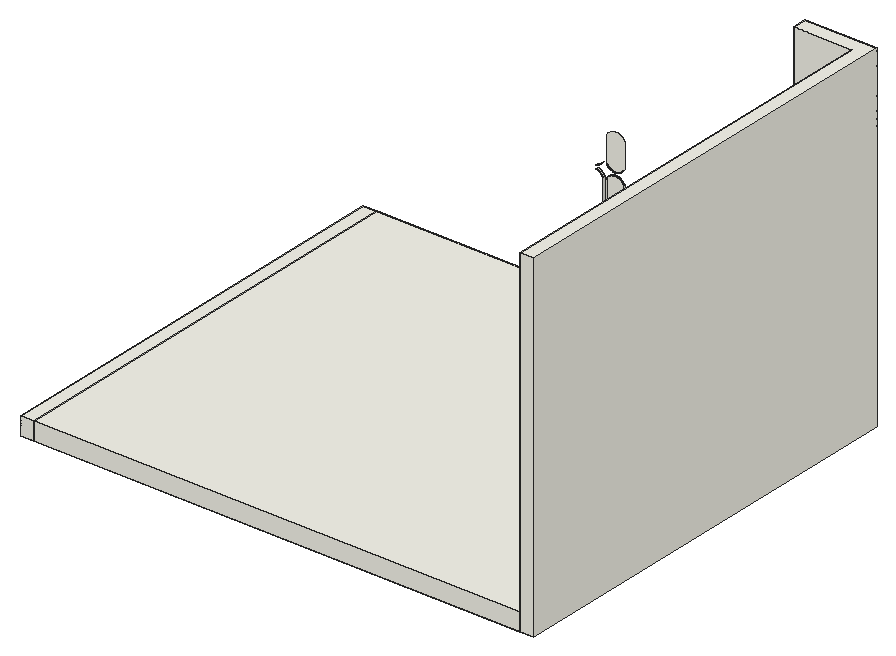
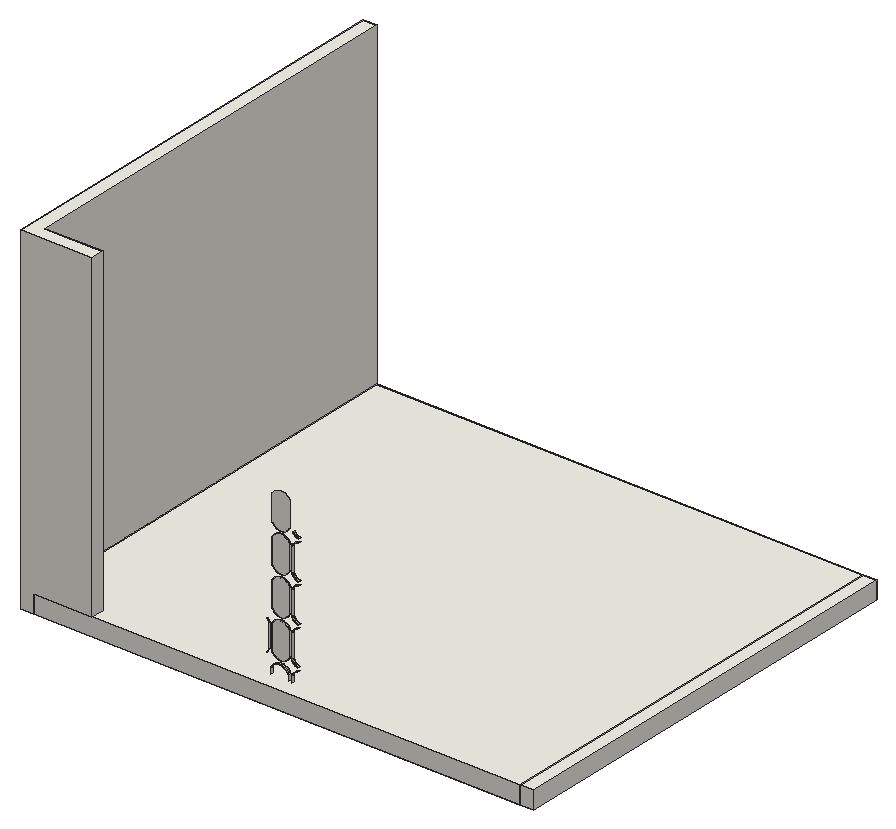
# SketchUp Ruby script. Lengths in inches.
U = 1.inch
M = Sketchup.active_model
def pt(a) = Geom::Point3d.new(a.map { |v| v * U })
def face(e, loops, mat)
  f = e.add_face(loops[0].map { |a| pt(a) })
  loops[1..].each { |l| e.add_face(l.map { |a| pt(a) }).erase! }
  f.material = f.back_material = mat if mat
  f
end
# faces: each face lists its corners as indices into pts; further lists are holes
def faces(e, pts, list, mat = nil) = list.each { |f| face(e, (f[0].is_a?(Array) ? f : [f]).map { |l| l.map { |i| pts[i] } }, mat) }
# xy, xz, yz: faces in a plane at the given z, y or x. An outline is a flat list of corners, or four numbers for a rectangle; further outlines are holes
def ring(l) = l.size == 4 ? [[l[0], l[1]], [l[2], l[1]], [l[2], l[3]], [l[0], l[3]]] : l.each_slice(2).to_a
def flat(e, list, mat, &to3) = list.each { |f| face(e, (f[0].is_a?(Array) ? f : [f]).map { |l| ring(l).map { |u, v| to3.(u, v) } }, mat) }
def xy(e, z, list, mat = nil) = flat(e, list, mat) { |x, y| [x, y, z] }
def xz(e, y, list, mat = nil) = flat(e, list, mat) { |x, z| [x, y, z] }
def yz(e, x, list, mat = nil) = flat(e, list, mat) { |y, z| [x, y, z] }
def lines(e, pts, list) = list.each { |a, b| e.add_line(pt(pts[a]), pt(pts[b])) }
# prism: a flat outline (further loops are holes) pulled along v
def prism(e, loops, v, mat = nil)
  f = face(e, loops, mat); d = Geom::Vector3d.new(v.map { |x| x * U })
  f.pushpull(f.normal.samedirection?(d) ? d.length : -d.length)
end
def box(e, o, s, mat = nil) = prism(e, [[o, [o[0] + s[0], o[1], o[2]], [o[0] + s[0], o[1] + s[1], o[2]], [o[0], o[1] + s[1], o[2]]]], [0, 0, s[2]], mat)
def at(x, y, z, deg = 0) = Geom::Transformation.translation(pt([x, y, z])) * Geom::Transformation.rotation(ORIGIN, Z_AXIS, deg.degrees)
def axes(o, x, y, z) = Geom::Transformation.new([*x, 0, *y, 0, *z, 0, *pt(o).to_a, 1])
def part(name) = M.definitions.add(name)
# library, detail: a bought-in or finely detailed component or shape, given as its bounding box
def library(name, o, s) = part(name).tap { |d| box(d.entities, o, s) }
def detail(e, o, s) = box(e.add_group.entities, o, s)
def put(e, d, t, mat = nil) = e.add_instance(d, t).tap { |i| i.material = mat if mat }
def group(e, t, mat = nil) = e.add_group.tap { |g| g.transformation = t; g.material = mat if mat }.entities
root = M.entities
M.materials.add("Tafisa-Gardenia-or-Gardenia-PM775-4K").color = [246, 245, 235]
xz(root,138.25,[[89.53,11,89.85,11.02,90.17,11.0625,90.48,11.14,90.78,11.25,91.07,11.38,91.35,11.55,91.61,11.73,91.84,11.95,92.0625,12.18,92.25,12.4375,92.42,12.71,92.5625,13,92.5625,21,92.42,21.29,92.25,21.5625,92.0625,21.82,91.84,22.05,91.61,22.27,91.35,22.45,91.07,22.62,90.78,22.75,90.48,22.86,90.17,22.9375,89.85,22.98,89.53,23,89.21,22.98,89.02,22.96,88.89,22.9375,88.58,22.86,88.28,22.75,87.99,22.62,87.72,22.45,87.46,22.27,87.22,22.05,87,21.82,86.81,21.5625,86.64,21.29,86.5,21,86.5,13,86.64,12.71,86.81,12.4375,87,12.18,87.22,11.95,87.46,11.73,87.72,11.55,87.99,11.38,88.28,11.25,88.58,11.14,88.89,11.0625,89.21,11.02],[89.53,24,89.85,24.02,90.17,24.0625,90.48,24.14,90.78,24.25,91.07,24.38,91.35,24.55,91.61,24.73,91.84,24.95,92.0625,25.18,92.25,25.4375,92.42,25.71,92.5625,26,92.5625,34,92.42,34.29,92.25,34.5625,92.0625,34.82,91.84,35.05,91.61,35.27,91.35,35.45,91.07,35.62,90.78,35.75,90.48,35.86,90.17,35.9375,89.85,35.98,89.53,36,89.21,35.98,89.02,35.96,88.89,35.9375,88.58,35.86,88.28,35.75,87.99,35.62,87.72,35.45,87.46,35.27,87.22,35.05,87,34.82,86.86,34.63,86.81,34.5625,86.64,34.29,86.5,34,86.5,26,86.64,25.71,86.81,25.4375,87,25.18,87.22,24.95,87.46,24.73,87.72,24.55,87.99,24.38,88.28,24.25,88.58,24.14,88.89,24.0625,89.02,24.04,89.21,24.02],[89.53,37,89.85,37.02,90.17,37.0625,90.48,37.14,90.78,37.25,91.07,37.38,91.35,37.55,91.61,37.73,91.84,37.95,92.0625,38.18,92.25,38.4375,92.42,38.71,92.5625,39,92.5625,47,92.42,47.29,92.25,47.5625,92.0625,47.82,91.84,48.05,91.61,48.27,91.35,48.45,91.07,48.62,90.78,48.75,90.48,48.86,90.17,48.9375,89.85,48.98,89.53,49,89.21,48.98,89.02,48.96,88.89,48.9375,88.58,48.86,88.28,48.75,87.99,48.62,87.72,48.45,87.46,48.27,87.22,48.05,87,47.82,86.81,47.5625,86.64,47.29,86.5,47,86.5,39,86.64,38.71,86.81,38.4375,87,38.18,87.22,37.95,87.46,37.73,87.72,37.55,87.99,37.38,88.28,37.25,88.58,37.14,88.89,37.0625,89.02,37.04,89.21,37.02],[89.53,50,89.85,50.02,90.17,50.0625,90.48,50.14,90.78,50.25,91.07,50.38,91.35,50.55,91.61,50.73,91.84,50.95,92.0625,51.18,92.25,51.4375,92.42,51.71,92.5625,52,92.5625,60,92.42,60.29,92.25,60.5625,92.0625,60.82,91.84,61.05,91.61,61.27,91.35,61.45,91.07,61.62,90.78,61.75,90.48,61.86,90.17,61.9375,89.85,61.98,89.53,62,89.21,61.98,89.02,61.96,88.89,61.9375,88.58,61.86,88.28,61.75,87.99,61.62,87.72,61.45,87.46,61.27,87.22,61.05,87,60.82,86.81,60.5625,86.64,60.29,86.5,60,86.5,52,86.64,51.71,86.81,51.4375,87,51.18,87.22,50.95,87.46,50.73,87.72,50.55,87.99,50.38,88.28,50.25,88.58,50.14,88.89,50.0625,89.02,50.04,89.21,50.02]],"Tafisa-Gardenia-or-Gardenia-PM775-4K")
yz(root,85.5,[[138,6,138.79,8],[138,13,138.79,21],[138,26,138.79,34],[138,39,138.79,47]])
yz(root,86.5,[[138,6,138.79,8]])
yz(root,86.5,[[138,13,138.25,21],[138,26,138.25,34],[138,39,138.25,47]],"Tafisa-Gardenia-or-Gardenia-PM775-4K")
yz(root,92.5625,[[138,6,138.79,8]])
yz(root,92.5625,[[138,13,138.25,21],[138,26,138.25,34],[138,39,138.25,47]],"Tafisa-Gardenia-or-Gardenia-PM775-4K")
yz(root,93.5625,[[138,13,138.25,21]],"Tafisa-Gardenia-or-Gardenia-PM775-4K")
p = [[85.36,138.79,8.29],[85.5,138.79,8],[85.5,138,8],[85.36,138,8.29],[86.5,138.79,8],[86.64,138.79,8.29],
  [86.64,138,8.29],[86.5,138,8],[92.42,138.79,8.29],[92.5625,138.79,8],[92.5625,138,8],[92.42,138,8.29],
  [85.2,138.79,8.56],[85.2,138,8.56],[86.81,138.79,8.5625],[86.81,138,8.5625],[92.25,138.79,8.5625],[92.25,138,8.5625],
  [85.01,138.79,8.82],[85.01,138,8.82],[87,138.79,8.82],[87,138,8.82],[92.0625,138.79,8.82],[92.0625,138,8.82],
  [84.79,138.79,9.05],[84.79,138,9.05],[87.22,138.79,9.05],[87.22,138,9.05],[91.84,138.79,9.05],[91.84,138,9.05],
  [84.56,138.79,9.26],[84.56,138,9.26],[87.46,138.79,9.27],[87.46,138,9.27],[91.61,138.79,9.27],[91.61,138,9.27],
  [84.3,138.79,9.45],[84.3,138,9.45],[87.72,138.79,9.45],[87.72,138,9.45],[91.35,138.79,9.45],[91.35,138,9.45],
  [84.03,138.79,9.62],[84.03,138,9.62],[87.99,138.79,9.62],[87.99,138,9.62],[91.07,138.79,9.62],[91.07,138,9.62],
  [83.74,138.79,9.75],[83.74,138,9.75],[88.28,138.79,9.75],[88.28,138,9.75],[90.78,138.79,9.75],[90.78,138,9.75],
  [83.44,138.79,9.86],[83.44,138,9.86],[88.58,138.79,9.86],[88.58,138,9.86],[90.48,138.79,9.86],[90.48,138,9.86],
  [88.89,138.79,9.9375],[88.89,138,9.9375],[89.21,138.79,9.98],[89.21,138,9.98],[89.85,138.79,9.98],[90.17,138.79,9.9375],
  [90.17,138,9.9375],[89.85,138,9.98],[89.53,138.79,10],[89.53,138,10],[88.89,138,11.0625],[89.21,138,11.02],
  [89.21,138.25,11.02],[88.89,138.25,11.0625],[89.53,138,11],[89.53,138.25,11],[89.85,138,11.02],[89.85,138.25,11.02],
  [90.17,138,11.0625],[90.17,138.25,11.0625],[83.74,138.79,11.25],[83.44,138.79,11.14],[83.44,138,11.14],[83.74,138,11.25],
  [88.28,138,11.25],[88.58,138,11.14],[88.58,138.25,11.14],[88.28,138.25,11.25],[90.48,138,11.14],[90.48,138.25,11.14],
  [90.78,138,11.25],[90.78,138.25,11.25],[84.03,138.79,11.38],[84.03,138,11.38],[87.99,138,11.38],[87.99,138.25,11.38],
  [91.07,138,11.38],[91.07,138.25,11.38],[84.3,138.79,11.55],[84.3,138,11.55],[87.72,138,11.55],[87.72,138.25,11.55],
  [91.35,138,11.55],[91.35,138.25,11.55],[84.56,138.79,11.74],[84.56,138,11.74],[87.46,138,11.73],[87.46,138.25,11.73],
  [91.61,138,11.73],[91.61,138.25,11.73],[84.79,138.79,11.95],[84.79,138,11.95],[87.22,138,11.95],[87.22,138.25,11.95],
  [91.84,138,11.95],[91.84,138.25,11.95],[85.01,138.79,12.18],[85.01,138,12.18],[87,138,12.18],[87,138.25,12.18],
  [92.0625,138,12.18],[92.0625,138.25,12.18],[94.04,138,12.19],[94.25,138,11.95],[94.25,138.25,11.95],[94.04,138.25,12.19],
  [85.2,138.79,12.44],[85.2,138,12.44],[86.81,138,12.4375],[86.81,138.25,12.4375],[92.25,138,12.4375],[92.25,138.25,12.4375],
  [93.86,138,12.44],[93.86,138.25,12.44],[85.36,138.79,12.71],[85.36,138,12.71],[86.64,138,12.71],[86.64,138.25,12.71],
  [92.42,138,12.71],[92.42,138.25,12.71],[93.7,138,12.71],[93.7,138.25,12.71],[85.5,138.79,13],[85.5,138,13],
  [86.5,138,13],[86.5,138.25,13],[92.5625,138,13],[92.5625,138.25,13],[93.5625,138,13],[93.5625,138.25,13],
  [85.36,138.79,21.29],[85.5,138.79,21],[85.5,138,21],[85.36,138,21.29],[86.64,138,21.29],[86.5,138,21],
  [86.5,138.25,21],[86.64,138.25,21.29],[92.5625,138,21],[92.42,138,21.29],[92.42,138.25,21.29],[92.5625,138.25,21],
  [93.7,138,21.29],[93.5625,138,21],[93.5625,138.25,21],[93.7,138.25,21.29],[85.2,138.79,21.56],[85.2,138,21.56],
  [86.81,138,21.5625],[86.81,138.25,21.5625],[92.25,138,21.5625],[92.25,138.25,21.5625],[93.86,138,21.56],[93.86,138.25,21.56],
  [85.01,138.79,21.82],[85.01,138,21.82],[87,138,21.82],[87,138.25,21.82],[92.0625,138,21.82],[92.0625,138.25,21.82],
  [94.04,138,21.81],[94.04,138.25,21.81],[84.79,138.79,22.05],[84.79,138,22.05],[87.22,138,22.05],[87.22,138.25,22.05],
  [91.84,138,22.05],[91.84,138.25,22.05],[94.25,138,22.05],[94.25,138.25,22.05],[84.56,138.79,22.26],[84.56,138,22.26],
  [87.46,138,22.27],[87.46,138.25,22.27],[91.61,138,22.27],[91.61,138.25,22.27],[84.3,138.79,22.45],[84.3,138,22.45],
  [87.72,138,22.45],[87.72,138.25,22.45],[91.35,138,22.45],[91.35,138.25,22.45],[84.03,138.79,22.62],[84.03,138,22.62],
  [87.99,138,22.62],[87.99,138.25,22.62],[91.07,138,22.62],[91.07,138.25,22.62],[83.74,138.79,22.75],[83.74,138,22.75],
  [88.28,138,22.75],[88.28,138.25,22.75],[90.78,138,22.75],[90.78,138.25,22.75],[83.44,138.79,22.86],[83.44,138,22.86],
  [88.58,138,22.86],[88.58,138.25,22.86],[90.48,138,22.86],[90.48,138.25,22.86],[88.89,138,22.9375],[88.89,138.25,22.9375],
  [89.02,138,22.96],[89.02,138.25,22.96],[90.17,138,22.9375],[89.85,138,22.98],[89.85,138.25,22.98],[90.17,138.25,22.9375],
  [89.21,138,22.98],[89.21,138.25,22.98],[89.53,138,23],[89.53,138.25,23],[88.89,138,24.0625],[89.02,138,24.04],
  [89.02,138.25,24.04],[88.89,138.25,24.0625],[89.21,138,24.02],[89.21,138.25,24.02],[89.53,138,24],[89.53,138.25,24],
  [89.85,138,24.02],[89.85,138.25,24.02],[90.17,138,24.0625],[90.17,138.25,24.0625],[83.44,138.79,24.14],[83.13,138.79,24.0625],
  [83.13,138,24.0625],[83.44,138,24.14],[83.74,138.79,24.25],[83.74,138,24.25],[88.28,138,24.25],[88.58,138,24.14],
  [88.58,138.25,24.14],[88.28,138.25,24.25],[90.48,138,24.14],[90.48,138.25,24.14],[90.78,138,24.25],[90.78,138.25,24.25],
  [84.03,138.79,24.38],[84.03,138,24.38],[87.99,138,24.38],[87.99,138.25,24.38],[91.07,138,24.38],[91.07,138.25,24.38],
  [84.3,138.79,24.55],[84.3,138,24.55],[87.72,138,24.55],[87.72,138.25,24.55],[91.35,138,24.55],[91.35,138.25,24.55],
  [84.56,138.79,24.74],[84.56,138,24.74],[87.46,138,24.73],[87.46,138.25,24.73],[91.61,138,24.73],[91.61,138.25,24.73],
  [84.79,138.79,24.95],[84.79,138,24.95],[87.22,138,24.95],[87.22,138.25,24.95],[91.84,138,24.95],[91.84,138.25,24.95],
  [85.01,138.79,25.18],[85.01,138,25.18],[87,138,25.18],[87,138.25,25.18],[92.0625,138,25.18],[92.0625,138.25,25.18],
  [85.2,138.79,25.44],[85.2,138,25.44],[86.81,138,25.4375],[86.81,138.25,25.4375],[92.25,138,25.4375],[92.25,138.25,25.4375],
  [85.36,138.79,25.71],[85.36,138,25.71],[86.64,138,25.71],[86.64,138.25,25.71],[92.42,138,25.71],[92.42,138.25,25.71],
  [85.5,138.79,26],[85.5,138,26],[86.5,138,26],[86.5,138.25,26],[92.5625,138,26],[92.5625,138.25,26],
  [85.36,138.79,34.29],[85.5,138.79,34],[85.5,138,34],[85.36,138,34.29],[86.64,138,34.29],[86.5,138,34],
  [86.5,138.25,34],[86.64,138.25,34.29],[92.5625,138,34],[92.42,138,34.29],[92.42,138.25,34.29],[92.5625,138.25,34],
  [85.2,138.79,34.56],[85.2,138,34.56],[86.81,138,34.5625],[86.81,138.25,34.5625],[92.25,138,34.5625],[92.25,138.25,34.5625],
  [85.01,138.79,34.82],[85.01,138,34.82],[86.86,138,34.63],[86.86,138.25,34.63],[87,138,34.82],[87,138.25,34.82],
  [92.0625,138,34.82],[92.0625,138.25,34.82],[84.79,138.79,35.05],[84.79,138,35.05],[87.22,138,35.05],[87.22,138.25,35.05],
  [91.84,138,35.05],[91.84,138.25,35.05],[84.56,138.79,35.26],[84.56,138,35.26],[87.46,138,35.27],[87.46,138.25,35.27],
  [91.61,138,35.27],[91.61,138.25,35.27],[84.3,138.79,35.45],[84.3,138,35.45],[87.72,138,35.45],[87.72,138.25,35.45],
  [91.35,138,35.45],[91.35,138.25,35.45],[84.03,138.79,35.62],[84.03,138,35.62],[87.99,138,35.62],[87.99,138.25,35.62],
  [91.07,138,35.62],[91.07,138.25,35.62],[83.74,138.79,35.75],[83.74,138,35.75],[88.28,138,35.75],[88.28,138.25,35.75],
  [90.78,138,35.75],[90.78,138.25,35.75],[83.44,138.79,35.86],[83.44,138,35.86],[88.58,138,35.86],[88.58,138.25,35.86],
  [90.48,138,35.86],[90.48,138.25,35.86],[83.13,138.79,35.9375],[83.13,138,35.9375],[88.89,138,35.9375],[88.89,138.25,35.9375],
  [89.02,138,35.96],[89.02,138.25,35.96],[90.17,138,35.9375],[89.85,138,35.98],[89.85,138.25,35.98],[90.17,138.25,35.9375],
  [89.21,138,35.98],[89.21,138.25,35.98],[89.53,138,36],[89.53,138.25,36],[88.89,138,37.0625],[89.02,138,37.04],
  [89.02,138.25,37.04],[88.89,138.25,37.0625],[89.21,138,37.02],[89.21,138.25,37.02],[89.53,138,37],[89.53,138.25,37],
  [89.85,138,37.02],[89.85,138.25,37.02],[90.17,138,37.0625],[90.17,138.25,37.0625],[83.44,138.79,37.14],[83.13,138.79,37.0625],
  [83.13,138,37.0625],[83.44,138,37.14],[83.74,138.79,37.25],[83.74,138,37.25],[88.28,138,37.25],[88.58,138,37.14],
  [88.58,138.25,37.14],[88.28,138.25,37.25],[90.48,138,37.14],[90.48,138.25,37.14],[90.78,138,37.25],[90.78,138.25,37.25],
  [84.03,138.79,37.38],[84.03,138,37.38],[87.99,138,37.38],[87.99,138.25,37.38],[91.07,138,37.38],[91.07,138.25,37.38],
  [84.3,138.79,37.55],[84.3,138,37.55],[87.72,138,37.55],[87.72,138.25,37.55],[91.35,138,37.55],[91.35,138.25,37.55],
  [84.46,138,37.66],[84.46,138.79,37.66],[87.46,138,37.73],[87.46,138.25,37.73],[91.61,138,37.73],[91.61,138.25,37.73],
  [84.56,138.79,37.74],[84.56,138,37.74],[84.79,138.79,37.95],[84.79,138,37.95],[87.22,138,37.95],[87.22,138.25,37.95],
  [91.84,138,37.95],[91.84,138.25,37.95],[85.01,138.79,38.18],[85.01,138,38.18],[87,138,38.18],[87,138.25,38.18],
  [92.0625,138,38.18],[92.0625,138.25,38.18],[85.2,138.79,38.44],[85.2,138,38.44],[86.81,138,38.4375],[86.81,138.25,38.4375],
  [92.25,138,38.4375],[92.25,138.25,38.4375],[85.36,138.79,38.71],[85.36,138,38.71],[86.64,138,38.71],[86.64,138.25,38.71],
  [92.42,138,38.71],[92.42,138.25,38.71],[85.5,138.79,39],[85.5,138,39],[86.5,138,39],[86.5,138.25,39],
  [92.5625,138,39],[92.5625,138.25,39],[85.36,138.79,47.29],[85.5,138.79,47],[85.5,138,47],[85.36,138,47.29],
  [86.64,138,47.29],[86.5,138,47],[86.5,138.25,47],[86.64,138.25,47.29],[92.5625,138,47],[92.42,138,47.29],
  [92.42,138.25,47.29],[92.5625,138.25,47],[85.2,138.79,47.56],[85.2,138,47.56],[86.81,138,47.5625],[86.81,138.25,47.5625],
  [92.25,138,47.5625],[92.25,138.25,47.5625],[85.01,138.79,47.82],[85.01,138,47.82],[87,138,47.82],[87,138.25,47.82],
  [92.0625,138,47.82],[92.0625,138.25,47.82],[84.79,138.79,48.05],[84.79,138,48.05],[87.22,138,48.05],[87.22,138.25,48.05],
  [91.84,138,48.05],[91.84,138.25,48.05],[84.56,138.79,48.26],[84.56,138,48.26],[87.46,138,48.27],[87.46,138.25,48.27],
  [91.61,138,48.27],[91.61,138.25,48.27],[84.3,138.79,48.45],[84.3,138,48.45],[87.72,138,48.45],[87.72,138.25,48.45],
  [91.35,138,48.45],[91.35,138.25,48.45],[84.03,138.79,48.62],[84.03,138,48.62],[87.99,138,48.62],[87.99,138.25,48.62],
  [91.07,138,48.62],[91.07,138.25,48.62],[83.74,138.79,48.75],[83.74,138,48.75],[88.28,138,48.75],[88.28,138.25,48.75],
  [90.78,138,48.75],[90.78,138.25,48.75],[83.44,138.79,48.86],[83.44,138,48.86],[88.58,138,48.86],[88.58,138.25,48.86],
  [90.48,138,48.86],[90.48,138.25,48.86],[83.13,138.79,48.9375],[83.13,138,48.9375],[88.89,138,48.9375],[88.89,138.25,48.9375],
  [89.02,138,48.96],[89.02,138.25,48.96],[90.17,138,48.9375],[89.85,138,48.98],[89.85,138.25,48.98],[90.17,138.25,48.9375],
  [89.21,138,48.98],[89.21,138.25,48.98],[89.53,138,49],[89.53,138.25,49],[88.89,138,50.0625],[89.02,138,50.04],
  [89.02,138.25,50.04],[88.89,138.25,50.0625],[89.21,138,50.02],[89.21,138.25,50.02],[89.53,138,50],[89.53,138.25,50],
  [89.85,138,50.02],[89.85,138.25,50.02],[90.17,138,50.0625],[90.17,138.25,50.0625],[83.44,138.79,50.14],[83.13,138.79,50.0625],
  [83.13,138,50.0625],[83.44,138,50.14],[83.74,138.79,50.25],[83.74,138,50.25],[88.28,138,50.25],[88.58,138,50.14],
  [88.58,138.25,50.14],[88.28,138.25,50.25],[90.48,138,50.14],[90.48,138.25,50.14],[90.78,138,50.25],[90.78,138.25,50.25],
  [84.03,138.79,50.38],[84.03,138,50.38],[87.99,138,50.38],[87.99,138.25,50.38],[91.07,138,50.38],[91.07,138.25,50.38],
  [84.3,138.79,50.55],[84.3,138,50.55],[87.72,138,50.55],[87.72,138.25,50.55],[91.35,138,50.55],[91.35,138.25,50.55],
  [84.56,138.79,50.74],[84.56,138,50.74],[87.46,138,50.73],[87.46,138.25,50.73],[91.61,138,50.73],[91.61,138.25,50.73],
  [84.79,138.79,50.95],[84.79,138,50.95],[87.22,138,50.95],[87.22,138.25,50.95],[91.84,138,50.95],[91.84,138.25,50.95],
  [85.01,138.79,51.18],[85.01,138,51.18],[87,138,51.18],[87,138.25,51.18],[92.0625,138,51.18],[92.0625,138.25,51.18],
  [85.2,138.79,51.44],[85.2,138,51.44],[86.81,138,51.4375],[86.81,138.25,51.4375],[92.25,138,51.4375],[92.25,138.25,51.4375]]
faces(root,p,[[0,1,2,3],[4,5,6,7],[8,9,10,11],[12,0,3,13],[5,14,15,6],[16,8,11,17],[18,12,13,19],[14,20,21,15],
  [22,16,17,23],[24,18,19,25],[20,26,27,21],[28,22,23,29],[30,24,25,31],[26,32,33,27],[34,28,29,35],[36,30,31,37],
  [32,38,39,33],[40,34,35,41],[42,36,37,43],[38,44,45,39],[46,40,41,47],[48,42,43,49],[44,50,51,45],[52,46,47,53],
  [54,48,49,55],[50,56,57,51],[58,52,53,59],[56,60,61,57],[60,62,63,61],[64,65,66,67],[65,58,59,66],[62,68,69,63],
  [68,64,67,69],[80,81,82,83],[92,80,83,93],[98,92,93,99],[104,98,99,105],[110,104,105,111],[116,110,111,117],[126,116,117,127],
  [134,126,127,135],[142,134,135,143],[150,151,152,153],[166,150,153,167],[174,166,167,175],[182,174,175,183],[190,182,183,191],[196,190,191,197],
  [202,196,197,203],[208,202,203,209],[214,208,209,215],[244,245,246,247],[248,244,247,249],[258,248,249,259],[264,258,259,265],[270,264,265,271],
  [276,270,271,277],[282,276,277,283],[288,282,283,289],[294,288,289,295],[300,294,295,301],[306,307,308,309],[318,306,309,319],[324,318,319,325],
  [332,324,325,333],[338,332,333,339],[344,338,339,345],[350,344,345,351],[356,350,351,357],[362,356,357,363],[368,362,363,369],[394,395,396,397],
  [398,394,397,399],[408,398,399,409],[414,408,409,415],[415,420,421,414],[426,421,420,427],[428,426,427,429],[434,428,429,435],[440,434,435,441],
  [446,440,441,447],[452,446,447,453],[458,459,460,461],[470,458,461,471],[476,470,471,477],[482,476,477,483],[488,482,483,489],[494,488,489,495],
  [500,494,495,501],[506,500,501,507],[512,506,507,513],[518,512,513,519],[544,545,546,547],[548,544,547,549],[558,548,549,559],[564,558,559,565],
  [570,564,565,571],[576,570,571,577],[582,576,577,583],[588,582,583,589]])
faces(root,p,[[70,71,72,73],[71,74,75,72],[74,76,77,75],[76,78,79,77],[84,85,86,87],[85,70,73,86],[78,88,89,79],[88,90,91,89],
  [94,84,87,95],[90,96,97,91],[100,94,95,101],[96,102,103,97],[106,100,101,107],[102,108,109,103],[112,106,107,113],[108,114,115,109],
  [118,112,113,119],[114,120,121,115],[122,123,124,125],[128,118,119,129],[120,130,131,121],[132,122,125,133],[136,128,129,137],[130,138,139,131],
  [140,132,133,141],[144,136,137,145],[138,146,147,139],[148,140,141,149],[154,155,156,157],[158,159,160,161],[162,163,164,165],[168,154,157,169],
  [159,170,171,160],[172,162,165,173],[176,168,169,177],[170,178,179,171],[180,172,173,181],[184,176,177,185],[178,186,187,179],[188,180,181,189],
  [192,184,185,193],[186,194,195,187],[198,192,193,199],[194,200,201,195],[204,198,199,205],[200,206,207,201],[210,204,205,211],[206,212,213,207],
  [216,210,211,217],[212,218,219,213],[220,216,217,221],[222,220,221,223],[224,225,226,227],[218,224,227,219],[228,222,223,229],[230,228,229,231],
  [225,230,231,226],[232,233,234,235],[233,236,237,234],[236,238,239,237],[238,240,241,239],[240,242,243,241],[250,251,252,253],[251,232,235,252],
  [242,254,255,243],[254,256,257,255],[260,250,253,261],[256,262,263,257],[266,260,261,267],[262,268,269,263],[272,266,267,273],[268,274,275,269],
  [278,272,273,279],[274,280,281,275],[284,278,279,285],[280,286,287,281],[290,284,285,291],[286,292,293,287],[296,290,291,297],[292,298,299,293],
  [302,296,297,303],[298,304,305,299],[310,311,312,313],[314,315,316,317],[320,310,313,321],[315,322,323,316],[326,320,321,327],[328,326,327,329],
  [322,330,331,323],[334,328,329,335],[330,336,337,331],[340,334,335,341],[336,342,343,337],[346,340,341,347],[342,348,349,343],[352,346,347,353],
  [348,354,355,349],[358,352,353,359],[354,360,361,355],[364,358,359,365],[360,366,367,361],[370,364,365,371],[372,370,371,373],[374,375,376,377],
  [366,374,377,367],[378,372,373,379],[380,378,379,381],[375,380,381,376],[382,383,384,385],[383,386,387,384],[386,388,389,387],[388,390,391,389],
  [390,392,393,391],[400,401,402,403],[401,382,385,402],[392,404,405,393],[404,406,407,405],[410,400,403,411],[406,412,413,407],[416,410,411,417],
  [412,418,419,413],[422,416,417,423],[418,424,425,419],[430,422,423,431],[424,432,433,425],[436,430,431,437],[432,438,439,433],[442,436,437,443],
  [438,444,445,439],[448,442,443,449],[444,450,451,445],[454,448,449,455],[450,456,457,451],[462,463,464,465],[466,467,468,469],[472,462,465,473],
  [467,474,475,468],[478,472,473,479],[474,480,481,475],[484,478,479,485],[480,486,487,481],[490,484,485,491],[486,492,493,487],[496,490,491,497],
  [492,498,499,493],[502,496,497,503],[498,504,505,499],[508,502,503,509],[504,510,511,505],[514,508,509,515],[510,516,517,511],[520,514,515,521],
  [522,520,521,523],[524,525,526,527],[516,524,527,517],[528,522,523,529],[530,528,529,531],[525,530,531,526],[532,533,534,535],[533,536,537,534],
  [536,538,539,537],[538,540,541,539],[540,542,543,541],[550,551,552,553],[551,532,535,552],[542,554,555,543],[554,556,557,555],[560,550,553,561],
  [556,562,563,557],[566,560,561,567],[562,568,569,563],[572,566,567,573],[568,574,575,569],[578,572,573,579],[574,580,581,575],[584,578,579,585],
  [580,586,587,581],[590,584,585,591],[586,592,593,587]],"Tafisa-Gardenia-or-Gardenia-PM775-4K")
g1 = group(root,at(4.5,0,0),"Tafisa-Gardenia-or-Gardenia-PM775-4K")
xy(g1,0,[[-4.5,0,0,144],[0,0,163.5,144],[163.5,0,168,144]])
xy(g1,5.88,[[-4.5,0,0,144],[0,0,163.5,0,163.5,139.5,144,139.5,144,144,0,144],[144,139.5,163.5,144]])
xy(g1,114,[[163.5,0,168,0,168,144,144,144,144,139.5,163.5,139.5]])
xz(g1,0,[[-4.5,0,0,5.88],[0,0,163.5,5.88],[163.5,0,168,114]])
xz(g1,139.5,[[144,5.88,163.5,114]])
xz(g1,144,[[-4.5,0,0,5.88],[0,0,163.5,5.88],[163.5,0,163.5,5.88,144,5.88,144,114,168,114,168,0]])
yz(g1,-4.5,[[0,0,144,5.88]])
yz(g1,0,[[0,0,144,5.88]])
yz(g1,144,[[139.5,5.88,144,114]])
yz(g1,163.5,[[0,0,144,5.88],[0,5.88,139.5,114]])
yz(g1,168,[[0,0,144,114]])
